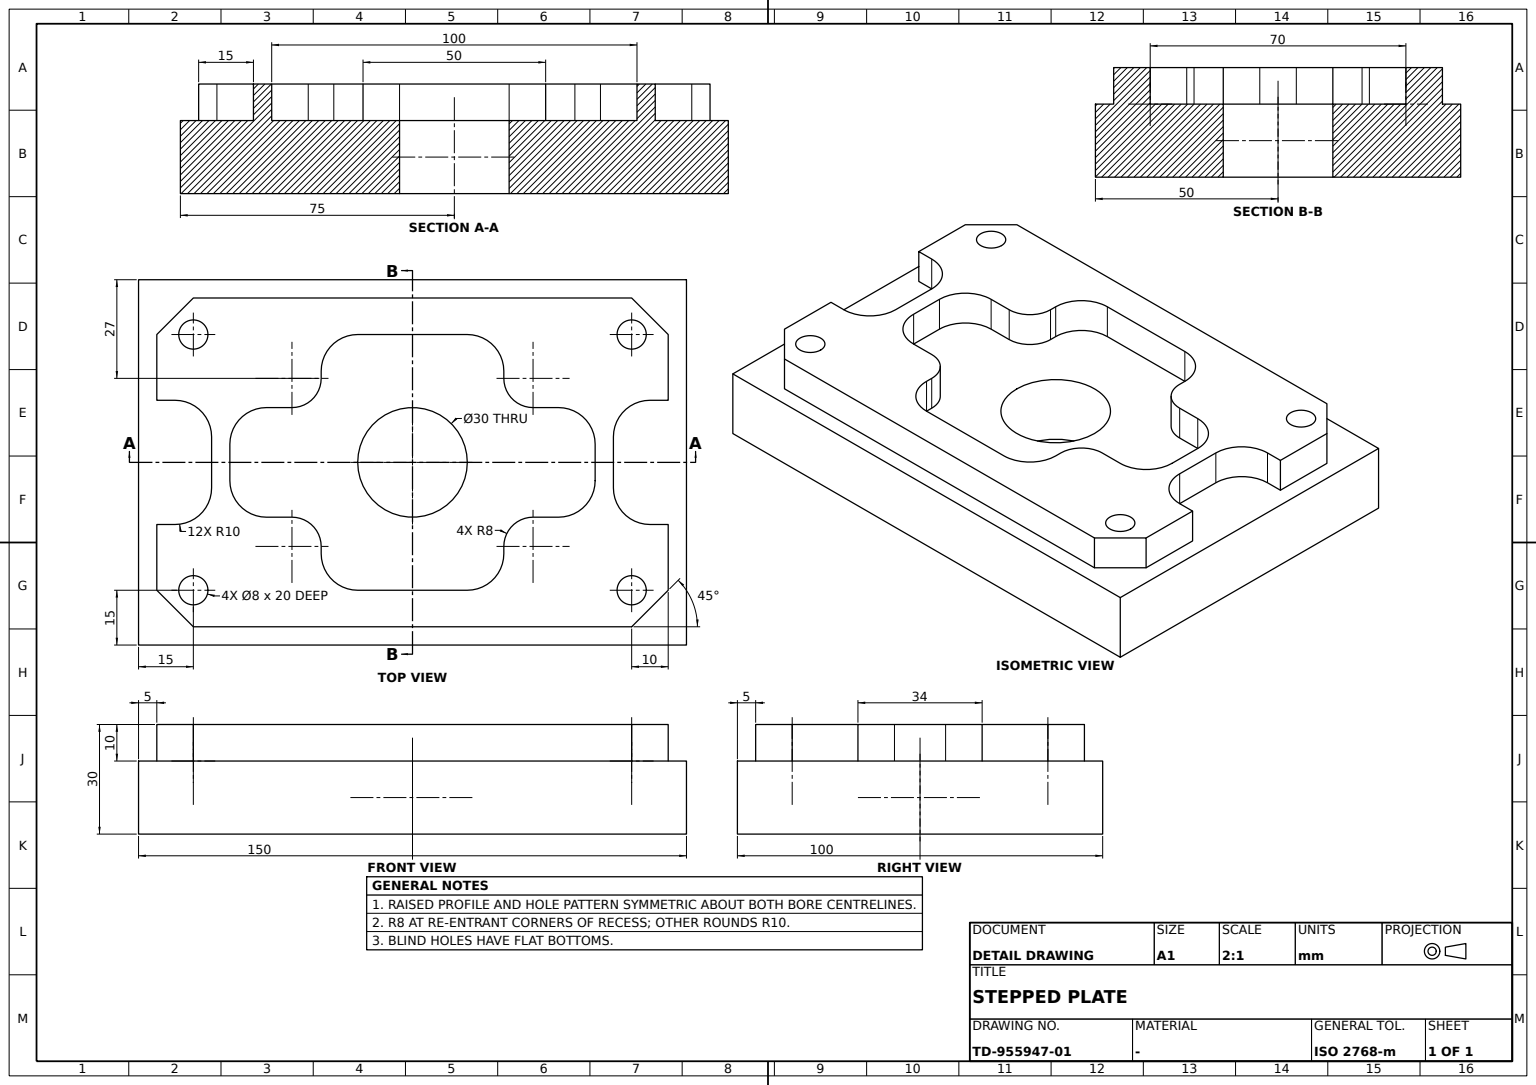
solid
v1 (50,5,-10)
v2 (50,5,0)
e1 v1 v2 LINE
v3 (50,-5,-10)
e2 v3 v1 LINE
v4 (50,-5,0)
e3 v3 v4 LINE
e4 v4 v2 LINE
face PLANE(AX(P(50,-5,-10),D(1,0,0),D(0,1,0))) rev [-e1 -e2 e3 e4]
v5 (55,7,-10)
v6 (65,17,-10)
e5 v5 v6 CIRCLE(AX(P(65,7,-10),D(0,0,1),D(1,0,0)),10) rev
v7 (65,17,0)
e6 v6 v7 LINE
v8 (55,7,0)
e7 v8 v7 CIRCLE(AX(P(65,7,0),D(0,0,-1),D(-1,0,0)),10)
e8 v5 v8 LINE
face CYL(AX(P(65,7,-5),D(0,0,-1),D(1,0,0)),10) rev [e5 e6 -e7 -e8]
v9 (-25,23,-10)
v10 (-33,15,-10)
e9 v9 v10 CIRCLE(AX(P(-33,23,-10),D(0,0,1),D(1,0,0)),8) rev
v11 (-25,23,0)
e10 v9 v11 LINE
v12 (-33,15,0)
e11 v11 v12 CIRCLE(AX(P(-33,23,0),D(0,0,-1),D(-1,0,0)),8)
e12 v10 v12 LINE
face CYL(AX(P(-33,23,-5),D(0,0,-1),D(1,0,0)),8) [-e9 e10 e11 -e12]
v13 (-70,17,-10)
v14 (-70,35,-10)
e13 v13 v14 LINE
v15 (-70,17,0)
e14 v13 v15 LINE
v16 (-70,35,0)
e15 v15 v16 LINE
e16 v14 v16 LINE
face PLANE(AX(P(-70,-45,-10),D(1,0,0),D(0,1,0))) rev [-e13 e14 e15 -e16]
v17 (55,-7,0)
e17 v8 v17 LINE
v18 (55,-7,-10)
e18 v18 v17 LINE
e19 v5 v18 LINE
face PLANE(AX(P(55,7,-10),D(-1,0,0),D(0,-1,0))) rev [e8 e17 -e18 -e19]
v19 (64,35,10)
e20 v19 v19 CIRCLE(AX(P(60,35,10),D(0,0,1),D(1,0,0)),4) rev
v20 (64,35,-10)
e21 v20 v20 CIRCLE(AX(P(60,35,-10),D(0,0,1),D(1,0,0)),4) rev
face CYL(AX(P(60,35,0),D(0,0,-1),D(1,0,0)),4) rev [-e20] [e21]
v21 (-65,17,0)
v22 (-55,7,0)
e22 v21 v22 CIRCLE(AX(P(-65,7,0),D(0,0,-1),D(-1,0,0)),10)
v23 (-65,17,-10)
e23 v23 v21 LINE
v24 (-55,7,-10)
e24 v23 v24 CIRCLE(AX(P(-65,7,-10),D(0,0,1),D(1,0,0)),10) rev
e25 v24 v22 LINE
face CYL(AX(P(-65,7,-5),D(0,0,-1),D(1,0,0)),10) rev [-e22 -e23 e24 e25]
v25 (-65,-17,0)
v26 (-70,-17,0)
e26 v25 v26 LINE
v27 (-65,-17,-10)
e27 v27 v25 LINE
v28 (-70,-17,-10)
e28 v27 v28 LINE
e29 v28 v26 LINE
face PLANE(AX(P(65,-17,-10),D(0,-1,0),D(1,0,0))) rev [-e26 -e27 e28 e29]
v29 (15,0,20)
e30 v29 v29 CIRCLE(AX(P(0,0,20),D(0,0,1),D(1,0,0)),15)
v30 (75,50,20)
v31 (75,-50,20)
e31 v30 v31 LINE
v32 (-75,50,20)
e32 v32 v30 LINE
v33 (-75,-50,20)
e33 v33 v32 LINE
e34 v31 v33 LINE
face PLANE(AX(P(0,0,20),D(0,0,1),D(1,0,0))) [-e30] [-e31 -e32 -e33 -e34]
v34 (60,-45,0)
v35 (-60,-45,0)
e35 v34 v35 LINE
v36 (-60,-45,-10)
e36 v35 v36 LINE
v37 (60,-45,-10)
e37 v37 v36 LINE
e38 v37 v34 LINE
face PLANE(AX(P(70,-45,-10),D(0,1,0),D(-1,0,0))) rev [e35 e36 -e37 e38]
v38 (-40,-15,-10)
v39 (-50,-5,-10)
e39 v38 v39 CIRCLE(AX(P(-40,-5,-10),D(0,0,1),D(1,0,0)),10) rev
v40 (-50,-5,0)
e40 v39 v40 LINE
v41 (-40,-15,0)
e41 v41 v40 CIRCLE(AX(P(-40,-5,0),D(0,0,-1),D(-1,0,0)),10)
e42 v38 v41 LINE
face CYL(AX(P(-40,-5,-5),D(0,0,-1),D(1,0,0)),10) rev [e39 e40 -e41 -e42]
v42 (33,-15,-10)
v43 (33,-15,0)
e43 v42 v43 LINE
v44 (40,-15,0)
e44 v43 v44 LINE
v45 (40,-15,-10)
e45 v45 v44 LINE
e46 v42 v45 LINE
face PLANE(AX(P(33,-15,-10),D(0,-1,0),D(1,0,0))) rev [e43 e44 -e45 -e46]
v46 (65,-17,-10)
v47 (70,-17,-10)
e47 v46 v47 LINE
v48 (65,-17,0)
e48 v46 v48 LINE
v49 (70,-17,0)
e49 v48 v49 LINE
e50 v47 v49 LINE
face PLANE(AX(P(65,-17,-10),D(0,-1,0),D(1,0,0))) rev [-e47 e48 e49 -e50]
v50 (-56,-35,10)
e51 v50 v50 CIRCLE(AX(P(-60,-35,10),D(0,0,1),D(1,0,0)),4) rev
v51 (-56,-35,-10)
e52 v51 v51 CIRCLE(AX(P(-60,-35,-10),D(0,0,1),D(1,0,0)),4) rev
face CYL(AX(P(-60,-35,0),D(0,0,-1),D(1,0,0)),4) rev [-e51] [e52]
v52 (-15,-35,-10)
v53 (15,-35,-10)
e53 v52 v53 LINE
v54 (-15,-35,0)
e54 v52 v54 LINE
v55 (15,-35,0)
e55 v54 v55 LINE
e56 v53 v55 LINE
face PLANE(AX(P(-15,-35,-10),D(0,-1,0),D(1,0,0))) rev [-e53 e54 e55 -e56]
v56 (64,-35,10)
e57 v56 v56 CIRCLE(AX(P(60,-35,10),D(0,0,1),D(1,0,0)),4) rev
face PLANE(AX(P(0,0,10),D(0,0,1),D(1,0,0))) rev [e57]
e58 v48 v17 CIRCLE(AX(P(65,-7,0),D(0,0,-1),D(-1,0,0)),10)
e59 v46 v18 CIRCLE(AX(P(65,-7,-10),D(0,0,1),D(1,0,0)),10) rev
face CYL(AX(P(65,-7,-5),D(0,0,-1),D(1,0,0)),10) rev [e18 -e58 -e48 e59]
v57 (25,25,-10)
v58 (25,25,0)
e60 v57 v58 LINE
v59 (15,35,0)
e61 v59 v58 CIRCLE(AX(P(15,25,0),D(0,0,-1),D(-1,0,0)),10)
v60 (15,35,-10)
e62 v60 v59 LINE
e63 v60 v57 CIRCLE(AX(P(15,25,-10),D(0,0,1),D(1,0,0)),10) rev
face CYL(AX(P(15,25,-5),D(0,0,-1),D(1,0,0)),10) rev [e60 -e61 -e62 e63]
v61 (25,-23,-10)
e64 v61 v42 CIRCLE(AX(P(33,-23,-10),D(0,0,1),D(1,0,0)),8) rev
v62 (25,-23,0)
e65 v61 v62 LINE
e66 v62 v43 CIRCLE(AX(P(33,-23,0),D(0,0,-1),D(-1,0,0)),8)
face CYL(AX(P(33,-23,-5),D(0,0,-1),D(1,0,0)),8) [-e64 e65 e66 -e43]
v63 (-15,0,0)
e67 v63 v63 CIRCLE(AX(P(0,0,0),D(0,0,-1),D(-1,0,0)),15)
v64 (-25,25,0)
e68 v64 v11 LINE
v65 (-15,35,0)
e69 v64 v65 CIRCLE(AX(P(-15,25,0),D(0,0,-1),D(-1,0,0)),10)
e70 v59 v65 LINE
v66 (25,23,0)
e71 v66 v58 LINE
v67 (33,15,0)
e72 v67 v66 CIRCLE(AX(P(33,23,0),D(0,0,-1),D(-1,0,0)),8)
v68 (40,15,0)
e73 v68 v67 LINE
e74 v68 v2 CIRCLE(AX(P(40,5,0),D(0,0,-1),D(-1,0,0)),10)
e75 v4 v44 CIRCLE(AX(P(40,-5,0),D(0,0,-1),D(-1,0,0)),10)
v69 (25,-25,0)
e76 v69 v62 LINE
e77 v69 v55 CIRCLE(AX(P(15,-25,0),D(0,0,-1),D(-1,0,0)),10)
v70 (-25,-25,0)
e78 v54 v70 CIRCLE(AX(P(-15,-25,0),D(0,0,-1),D(-1,0,0)),10)
v71 (-25,-23,0)
e79 v71 v70 LINE
v72 (-33,-15,0)
e80 v72 v71 CIRCLE(AX(P(-33,-23,0),D(0,0,-1),D(-1,0,0)),8)
e81 v41 v72 LINE
v73 (-50,5,0)
e82 v73 v40 LINE
v74 (-40,15,0)
e83 v73 v74 CIRCLE(AX(P(-40,5,0),D(0,0,-1),D(-1,0,0)),10)
e84 v12 v74 LINE
face PLANE(AX(P(0,0,0),D(0,0,-1),D(1,0,0))) [-e67] [-e11 -e68 e69 -e70 e61 -e71 -e72 -e73 e74 -e4 e75 -e44 -e66 -e76 e77 -e55 e78 -e79 -e80 -e81 e41 -e82 e83 -e84]
v75 (-50,5,-10)
e85 v75 v39 LINE
e86 v75 v73 LINE
face PLANE(AX(P(-50,5,-10),D(-1,0,0),D(0,-1,0))) rev [e82 -e40 -e85 e86]
face PLANE(AX(P(0,0,10),D(0,0,1),D(1,0,0))) rev [e51]
face CYL(AX(P(0,0,10.66),D(0,0,-1),D(1,0,0)),15) rev [e67] [e30]
v76 (33,15,-10)
e87 v76 v67 LINE
v77 (40,15,-10)
e88 v77 v76 LINE
e89 v77 v68 LINE
face PLANE(AX(P(-33,15,-10),D(0,1,0),D(-1,0,0))) rev [e73 -e87 -e88 e89]
v78 (-75,50,0)
e90 v32 v78 LINE
v79 (-75,-50,0)
e91 v79 v78 LINE
e92 v33 v79 LINE
face PLANE(AX(P(-75,-50,0),D(-1,0,0),D(0,1,0))) [e33 e90 -e91 -e92]
v80 (70,35,-10)
v81 (70,17,-10)
e93 v80 v81 LINE
v82 (70,35,0)
e94 v82 v80 LINE
v83 (70,17,0)
e95 v82 v83 LINE
e96 v81 v83 LINE
face PLANE(AX(P(70,45,-10),D(-1,0,0),D(0,-1,0))) rev [-e93 -e94 e95 -e96]
e97 v15 v21 LINE
e98 v13 v23 LINE
face PLANE(AX(P(70,17,-10),D(0,1,0),D(-1,0,0))) rev [e23 -e97 -e14 e98]
v84 (-40,15,-10)
e99 v75 v84 CIRCLE(AX(P(-40,5,-10),D(0,0,1),D(1,0,0)),10) rev
e100 v84 v74 LINE
face CYL(AX(P(-40,5,-5),D(0,0,-1),D(1,0,0)),10) rev [-e83 -e86 e99 e100]
v85 (-70,-35,0)
e101 v85 v35 LINE
v86 (-70,-35,-10)
e102 v85 v86 LINE
e103 v86 v36 LINE
face PLANE(AX(P(-60,-45,2),D(0.707106781,0.707106781,0),D(0,0,-1))) rev [-e101 e102 e103 -e36]
e104 v10 v84 LINE
face PLANE(AX(P(-33,15,-10),D(0,1,0),D(-1,0,0))) rev [-e104 e12 e84 -e100]
v87 (-56,35,10)
e105 v87 v87 CIRCLE(AX(P(-60,35,10),D(0,0,1),D(1,0,0)),4) rev
face PLANE(AX(P(0,0,10),D(0,0,1),D(1,0,0))) rev [e105]
v88 (75,50,0)
e106 v30 v88 LINE
e107 v78 v88 LINE
face PLANE(AX(P(-75,50,0),D(0,1,0),D(1,0,0))) [-e90 e32 e106 -e107]
v89 (25,23,-10)
e108 v89 v66 LINE
e109 v76 v89 CIRCLE(AX(P(33,23,-10),D(0,0,1),D(1,0,0)),8) rev
face CYL(AX(P(33,23,-5),D(0,0,-1),D(1,0,0)),8) [e87 e72 -e108 -e109]
v90 (-55,-7,0)
e110 v90 v25 CIRCLE(AX(P(-65,-7,0),D(0,0,-1),D(-1,0,0)),10)
v91 (-55,-7,-10)
e111 v91 v90 LINE
e112 v91 v27 CIRCLE(AX(P(-65,-7,-10),D(0,0,1),D(1,0,0)),10) rev
face CYL(AX(P(-65,-7,-5),D(0,0,-1),D(1,0,0)),10) rev [-e110 -e111 e112 e27]
v92 (60,45,0)
v93 (60,45,-10)
e113 v92 v93 LINE
e114 v82 v92 LINE
e115 v93 v80 LINE
face PLANE(AX(P(60,45,2),D(-0.707106781,-0.707106781,0),D(0,0,-1))) rev [-e113 -e114 e94 -e115]
e116 v83 v7 LINE
e117 v81 v6 LINE
face PLANE(AX(P(70,17,-10),D(0,1,0),D(-1,0,0))) rev [e96 e116 -e6 -e117]
v94 (-25,-23,-10)
e118 v94 v71 LINE
v95 (-33,-15,-10)
e119 v95 v94 CIRCLE(AX(P(-33,-23,-10),D(0,0,1),D(1,0,0)),8) rev
e120 v95 v72 LINE
face CYL(AX(P(-33,-23,-5),D(0,0,-1),D(1,0,0)),8) [-e118 -e119 e120 e80]
v96 (70,-35,-10)
v97 (70,-35,0)
e121 v96 v97 LINE
e122 v34 v97 LINE
e123 v96 v37 LINE
face PLANE(AX(P(60,-45,-12),D(-0.707106781,0.707106781,0),D(0,0,1))) rev [e121 -e122 -e38 -e123]
v98 (-60,45,-10)
e124 v98 v93 LINE
v99 (-60,45,0)
e125 v98 v99 LINE
e126 v99 v92 LINE
face PLANE(AX(P(-70,45,-10),D(0,-1,0),D(1,0,0))) rev [-e124 e125 e126 e113]
v100 (-25,-25,-10)
e127 v52 v100 CIRCLE(AX(P(-15,-25,-10),D(0,0,1),D(1,0,0)),10) rev
e128 v100 v70 LINE
face CYL(AX(P(-15,-25,-5),D(0,0,-1),D(1,0,0)),10) rev [-e54 e127 e128 -e78]
v101 (-25,25,-10)
e129 v101 v9 LINE
e130 v38 v95 LINE
e131 v94 v100 LINE
v102 (25,-25,-10)
e132 v102 v53 CIRCLE(AX(P(15,-25,-10),D(0,0,1),D(1,0,0)),10) rev
e133 v102 v61 LINE
e134 v3 v45 CIRCLE(AX(P(40,-5,-10),D(0,0,1),D(1,0,0)),10) rev
e135 v77 v1 CIRCLE(AX(P(40,5,-10),D(0,0,1),D(1,0,0)),10) rev
e136 v89 v57 LINE
v103 (-15,35,-10)
e137 v60 v103 LINE
e138 v101 v103 CIRCLE(AX(P(-15,25,-10),D(0,0,1),D(1,0,0)),10) rev
e139 v24 v91 LINE
e140 v14 v98 LINE
e141 v47 v96 LINE
e142 v86 v28 LINE
v104 (-56,35,-10)
e143 v104 v104 CIRCLE(AX(P(-60,35,-10),D(0,0,1),D(1,0,0)),4) rev
v105 (64,-35,-10)
e144 v105 v105 CIRCLE(AX(P(60,-35,-10),D(0,0,1),D(1,0,0)),4) rev
face PLANE(AX(P(0,0,-10),D(0,0,1),D(1,0,0))) rev [e129 e9 e104 -e99 e85 -e39 e130 e119 e131 -e127 e53 -e132 e133 e64 e46 -e134 e2 -e135 e88 e109 e136 -e63 e137 -e138] [-e139 -e24 -e98 e13 e140 e124 e115 e93 e117 -e5 e19 -e59 e47 e141 e123 e37 -e103 e142 -e28 -e112] [-e52] [-e21] [-e143] [-e144]
e145 v102 v69 LINE
face CYL(AX(P(15,-25,-5),D(0,0,-1),D(1,0,0)),10) rev [e132 e56 -e77 -e145]
face PLANE(AX(P(25,-25,-10),D(1,0,0),D(0,1,0))) rev [e71 -e60 -e136 e108]
face PLANE(AX(P(0,0,10),D(0,0,1),D(1,0,0))) rev [e20]
v106 (75,-50,0)
e146 v31 v106 LINE
e147 v88 v106 LINE
face PLANE(AX(P(75,50,0),D(1,0,0),D(0,-1,0))) [e146 -e147 -e106 e31]
e148 v106 v79 LINE
face PLANE(AX(P(75,-50,0),D(0,-1,0),D(-1,0,0))) [e92 -e148 -e146 e34]
e149 v85 v26 LINE
e150 v49 v97 LINE
e151 v16 v99 LINE
e152 v22 v90 LINE
face PLANE(AX(P(0,0,0),D(0,0,-1),D(1,0,0))) [-e149 e101 -e35 e122 -e150 -e49 e58 -e17 e7 -e116 -e95 e114 -e126 -e151 -e15 e97 e22 e152 e110 e26] [e147 e148 e91 e107]
face PLANE(AX(P(33,-15,-10),D(0,-1,0),D(1,0,0))) rev [e42 e81 -e120 -e130]
face CYL(AX(P(40,-5,-5),D(0,0,-1),D(1,0,0)),10) rev [e45 -e75 -e3 e134]
e153 v101 v64 LINE
face PLANE(AX(P(-25,-23,-10),D(-1,0,0),D(0,-1,0))) rev [-e10 -e129 e153 e68]
e154 v103 v65 LINE
face PLANE(AX(P(15,35,-10),D(0,1,0),D(-1,0,0))) rev [-e137 e62 e70 -e154]
face CYL(AX(P(-15,25,-5),D(0,0,-1),D(1,0,0)),10) rev [e154 -e69 -e153 e138]
face CYL(AX(P(60,-35,0),D(0,0,-1),D(1,0,0)),4) rev [-e57] [e144]
face CYL(AX(P(-60,35,0),D(0,0,-1),D(1,0,0)),4) rev [e143] [-e105]
face PLANE(AX(P(-25,-23,-10),D(-1,0,0),D(0,-1,0))) rev [e118 e79 -e128 -e131]
face PLANE(AX(P(25,-25,-10),D(1,0,0),D(0,1,0))) rev [e145 e76 -e65 -e133]
face PLANE(AX(P(-70,-45,-10),D(1,0,0),D(0,1,0))) rev [e149 -e29 -e142 -e102]
face PLANE(AX(P(-55,7,-10),D(-1,0,0),D(0,-1,0))) [e111 -e152 -e25 e139]
face PLANE(AX(P(-60,45,-12),D(0.707106781,-0.707106781,0),D(0,0,1))) rev [-e140 e16 e151 -e125]
face CYL(AX(P(40,5,-5),D(0,0,-1),D(1,0,0)),10) rev [-e89 e135 e1 -e74]
face PLANE(AX(P(70,45,-10),D(-1,0,0),D(0,-1,0))) rev [e150 -e121 -e141 e50]
